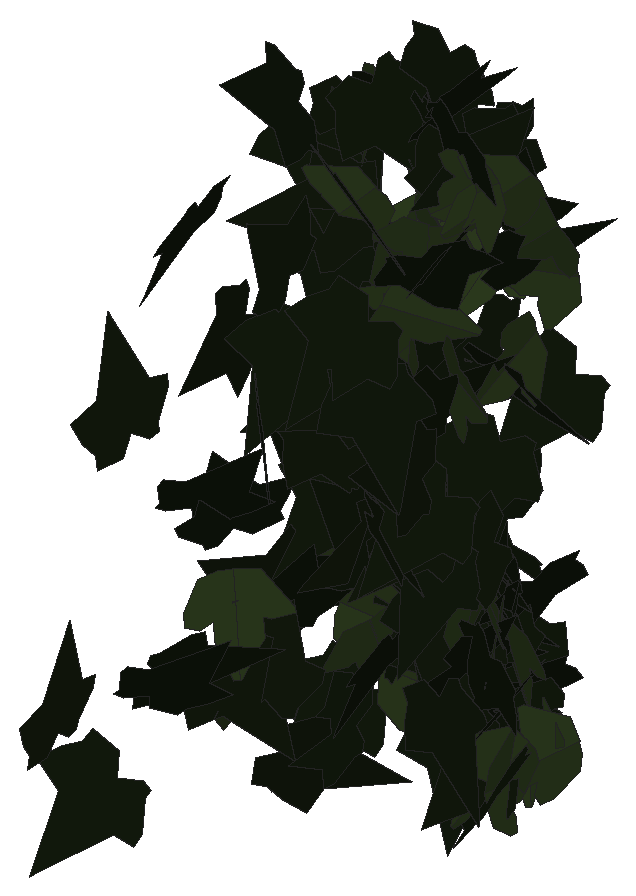
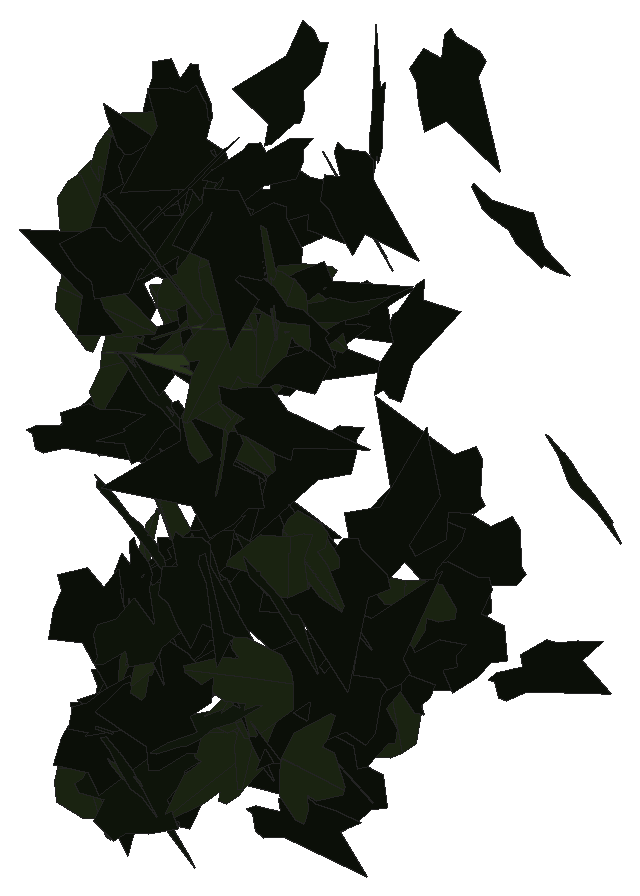
# SketchUp Ruby script. Lengths in inches.
U = 1.inch
M = Sketchup.active_model
def pt(a) = Geom::Point3d.new(a.map { |v| v * U })
def face(e, loops, mat)
  f = e.add_face(loops[0].map { |a| pt(a) })
  loops[1..].each { |l| e.add_face(l.map { |a| pt(a) }).erase! }
  f.material = f.back_material = mat if mat
  f
end
# faces: each face lists its corners as indices into pts; further lists are holes
def faces(e, pts, list, mat = nil) = list.each { |f| face(e, (f[0].is_a?(Array) ? f : [f]).map { |l| l.map { |i| pts[i] } }, mat) }
# xy, xz, yz: faces in a plane at the given z, y or x. An outline is a flat list of corners, or four numbers for a rectangle; further outlines are holes
def ring(l) = l.size == 4 ? [[l[0], l[1]], [l[2], l[1]], [l[2], l[3]], [l[0], l[3]]] : l.each_slice(2).to_a
def flat(e, list, mat, &to3) = list.each { |f| face(e, (f[0].is_a?(Array) ? f : [f]).map { |l| ring(l).map { |u, v| to3.(u, v) } }, mat) }
def xy(e, z, list, mat = nil) = flat(e, list, mat) { |x, y| [x, y, z] }
def xz(e, y, list, mat = nil) = flat(e, list, mat) { |x, z| [x, y, z] }
def yz(e, x, list, mat = nil) = flat(e, list, mat) { |y, z| [x, y, z] }
def lines(e, pts, list) = list.each { |a, b| e.add_line(pt(pts[a]), pt(pts[b])) }
# prism: a flat outline (further loops are holes) pulled along v
def prism(e, loops, v, mat = nil)
  f = face(e, loops, mat); d = Geom::Vector3d.new(v.map { |x| x * U })
  f.pushpull(f.normal.samedirection?(d) ? d.length : -d.length)
end
def box(e, o, s, mat = nil) = prism(e, [[o, [o[0] + s[0], o[1], o[2]], [o[0] + s[0], o[1] + s[1], o[2]], [o[0], o[1] + s[1], o[2]]]], [0, 0, s[2]], mat)
def at(x, y, z, deg = 0) = Geom::Transformation.translation(pt([x, y, z])) * Geom::Transformation.rotation(ORIGIN, Z_AXIS, deg.degrees)
def axes(o, x, y, z) = Geom::Transformation.new([*x, 0, *y, 0, *z, 0, *pt(o).to_a, 1])
def part(name) = M.definitions.add(name)
# library, detail: a bought-in or finely detailed component or shape, given as its bounding box
def library(name, o, s) = part(name).tap { |d| box(d.entities, o, s) }
def detail(e, o, s) = box(e.add_group.entities, o, s)
def put(e, d, t, mat = nil) = e.add_instance(d, t).tap { |i| i.material = mat if mat }
def group(e, t, mat = nil) = e.add_group.tap { |g| g.transformation = t; g.material = mat if mat }.entities
root = M.entities
M.materials.add("efeu1").color = [18, 25, 13]
M.materials.add("efeu2").color = [43, 57, 29]
c1 = part("ivyleaf_9")
p = [[1.54,2.16,1.25],[1.36,2.04,1.19],[-0.21,0.99,0.68],[-0.71,1.11,0.82],[-0.85,0.86,0.67],[-0.8,0.17,0.21],
  [-0.9,-0.01,0.1],[-0.67,-0.16,-0.02],[-0.08,-0.08,-0.05],[-0.03,-0.6,-0.4],[0.65,-0.88,-0.66],[0.83,-0.6,-0.49],
  [1.29,-0.42,-0.43],[1.8125,-0.07,-0.26],[1.21,0.44,0.15]]
faces(c1.entities,p,[[0,1,2,3,4,5,6,7,8,9,10,11,12,13,14]],"efeu1")
c2 = part("ivyleaf_10")
p = [[0,0.5,-0.03],[-0.0625,2.02,-0.43],[-0.19,2.01,-0.46],[-0.54,1.05,-0.29],[-0.52,0.625,-0.18],[-0.83,0.76,-0.28],
  [-1.16,0.64,-0.33],[-1.15,0.33,-0.24],[-0.77,-0.39,0.02],[-0.3,-0.51,0.16],[0.04,-0.48,0.23],[-0.02,2.01,-0.4375],
  [-0.06,2.01,-0.43],[0.04,-0.49,0.23],[0.67,-0.49,0.14],[1.38,0.36,-0.2],[1.375,0.51,-0.24],[0.81,0.65,-0.19],
  [0.62,0.59,-0.15],[0.6,1.09,-0.28],[0.5,1.23,-0.31]]
faces(c2.entities,p,[[0,1,2,3,4,5,6,7,8,9,10],[11,12,0,13,14,15,16,17,18,19,20]],"efeu2")
put(root,c1,axes([49.99,215.57,235.71],[-0.39967,0.22054,-0.20402],[-0.18022,0.09569,0.45647],[0.24039,0.43841,0.003]))
put(root,c1,axes([52.22,216.5,239.71],[-0.02606,0.03411,0.49815],[0.07343,-0.49315,0.0376],[0.49389,0.07512,0.02069]))
put(root,c1,axes([50.27,216.52,239.3],[-0.47515,0.08384,-0.13118],[-0.13302,0.00028,0.48198],[0.08089,0.49292,0.02204]))
put(root,c1,axes([49.53,217.14,234.17],[-0.31074,-0.35872,0.15736],[-0.10655,-0.11589,-0.47457],[0.37695,-0.32847,-0.00442]))
put(root,c1,axes([50.48,217.46,241.78],[-0.23217,0.35561,-0.26389],[0.13647,-0.226,-0.42462],[-0.42127,-0.2692,0.00789]))
put(root,c1,axes([49.88,217.44,235.3],[0.37642,0.32647,-0.04159],[0.02869,0.03039,0.49825],[0.32785,-0.37749,0.00415]))
put(root,c1,axes([49.58,218.01,235.21],[0.02408,0.29514,-0.40288],[0.03938,0.40097,0.29609],[0.49787,-0.04599,-0.00394]))
put(root,c1,axes([51.875,218.76,240.21],[-0.40406,-0.29221,0.03674],[-0.03289,-0.01721,-0.49862],[0.29267,-0.40536,-0.00532]))
put(root,c1,axes([52.09,218.73,239.49],[-0.02694,-0.47008,-0.16822],[0.03156,0.16653,-0.4704],[0.49828,-0.03596,0.0207]))
put(root,c1,axes([49.41,218.78,237],[0.38796,0.31541,0.00014],[-0.00169,0.00186,0.49999],[0.31541,-0.38796,0.0025]))
put(root,c1,axes([51.34,218.98,241.81],[0.31594,-0.31123,0.23091],[0.16229,-0.16428,-0.44348],[0.35191,0.35517,-0.00279]))
put(root,c1,axes([50.64,219.21,239.34],[-0.27085,-0.41475,0.06801],[-0.03151,-0.06064,-0.49531],[0.4191,-0.27259,0.00671]))
put(root,c1,axes([49.67,219.32,239.28],[0.00942,-0.16959,-0.47027],[0.31624,-0.36226,0.13697],[-0.38718,-0.30001,0.10044]))
put(root,c1,axes([50.76,218.77,240.5],[-0.16989,0.28729,0.37229],[-0.19955,0.31439,-0.33367],[-0.42581,-0.26196,0.00784]))
put(root,c2,axes([49.76,219.04,235.87],[0.407,0.28424,0.05961],[0.05015,0.03231,-0.49643],[-0.28607,0.41007,-0.00221]))
put(root,c1,axes([49.73,218.95,235.04],[0.03855,-0.32128,-0.38117],[0.01394,0.38285,-0.32129],[0.49832,0.01415,0.03848]))
put(root,c1,axes([52.12,219.47,238],[-0.06064,-0.06194,0.49243],[-0.20002,-0.45097,-0.08135],[0.45422,-0.20686,0.02991]))
put(root,c1,axes([49.55,219.3125,236.56],[0.30021,0.20075,0.34579],[-0.28282,-0.19905,0.3611],[0.28264,-0.41241,-0.00596]))
put(root,c2,axes([49.65,219.38,234.29],[0.02323,-0.49628,-0.05623],[0.00614,-0.056,0.49682],[-0.49942,-0.02378,0.0035]))
put(root,c1,axes([50.09,219.21,234.6],[-0.45453,0.0486,0.20258],[0.20123,-0.02344,0.45712],[0.05393,0.49708,0.00175]))
put(root,c1,axes([51.67,219.27,237.35],[0.41217,-0.17687,-0.22098],[-0.18981,0.11686,-0.44757],[0.20997,0.45284,0.02919]))
put(root,c1,axes([51,219.74,238.76],[-0.32371,-0.22221,0.30957],[-0.26412,-0.16196,-0.39244],[0.27468,-0.4176,-0.01253]))
put(root,c1,axes([51.67,219.51,235.67],[-0.21928,0.35771,-0.27195],[0.12805,-0.24032,-0.41935],[-0.43072,-0.25355,0.01378]))
put(root,c1,axes([52.16,219.8,237.59],[-0.36068,-0.33052,0.10327],[-0.07652,-0.06935,-0.48922],[0.33772,-0.36871,-0.00056]))
put(root,c1,axes([52.24,219.77,236.86],[-0.42698,-0.17845,-0.18931],[0.19423,0.02341,-0.46014],[0.17309,-0.46648,0.04933]))
put(root,c1,axes([49.86,219.67,235.33],[0.35674,0.31707,0.14902],[-0.11277,-0.09743,0.47727],[0.33169,-0.37413,0.00199]))
put(root,c1,axes([49.65,220,235.33],[0.05053,0.04046,0.49579],[-0.36123,-0.33963,0.06453],[0.34199,-0.36471,-0.00509]))
put(root,c1,axes([50.97,219.68,234.27],[-0.4208,0.24404,0.11564],[-0.10703,0.04586,-0.48625],[-0.24793,-0.43398,0.01364]))
put(root,c1,axes([50.17,219.48,233.73],[0.11932,0.13314,-0.46694],[0.22307,0.41205,0.1745],[0.43128,-0.24997,0.03893]))
put(root,c1,axes([51.97,219.96,237.24],[-0.49563,-0.06499,0.01127],[-0.01088,-0.00367,-0.49987],[0.06505,-0.49574,0.00222]))
put(root,c1,axes([51.45,220.13,236.82],[-0.07828,-0.03733,-0.49242],[0.01006,-0.49859,0.0362],[-0.49373,-0.00424,0.07881]))
put(root,c1,axes([51.17,219.64,236.79],[-0.28381,0.04697,-0.40896],[-0.41137,-0.01428,0.28385],[0.01498,0.49758,0.04675]))
put(root,c1,axes([52.07,219.93,234.85],[0.17337,-0.45792,-0.10124],[-0.03661,0.09439,-0.48964],[0.46755,0.17719,-0.0008]))
put(root,c1,axes([52.73,219.98,237.13],[-0.49394,0.07522,-0.01909],[0.01888,-0.00279,-0.49964],[-0.07527,-0.4943,-0.00008]))
put(root,c2,axes([52.0625,220.16,238.91],[-0.07368,-0.00952,0.49445],[0.47229,-0.14961,0.0675],[0.14666,0.477,0.03104]))
put(root,c1,axes([51.78,219.67,238.54],[0.1472,0.037,0.47641],[0.35605,0.32397,-0.13517],[-0.31869,0.37904,0.06903]))
put(root,c1,axes([50.36,219.93,237.98],[0.06698,-0.32711,-0.37217],[-0.04897,0.36935,-0.33344],[0.49307,0.08112,0.01744]))
put(root,c1,axes([49.59,219.68,234.74],[0.0962,0.1016,0.48002],[0.25664,0.40649,-0.13747],[-0.41819,0.27284,0.02606]))
put(root,c1,axes([49.73,220.2,241.74],[-0.11921,0.07273,-0.4801],[-0.46417,-0.16227,0.09067],[-0.14262,0.46731,0.1062]))
put(root,c1,axes([51.73,220.04,240.45],[0.26999,0.41183,-0.08662],[-0.05092,-0.07019,-0.49242],[-0.41775,0.27472,0.00404]))
put(root,c1,axes([52.59,220.16,235.5],[0.21252,0.03055,-0.45156],[-0.44708,-0.06345,-0.2147],[-0.07042,0.49502,0.00034]))
put(root,c1,axes([52.73,220.09,233.81],[-0.20504,0.4481,0.08467],[-0.05113,0.06966,-0.49248],[-0.45315,-0.21061,0.01725]))
put(root,c1,axes([52.09,220.21,242.14],[0.29541,0.04984,-0.40031],[-0.39674,-0.05391,-0.29949],[-0.07302,0.49458,0.0077]))
put(root,c2,axes([52.32,220.34,241.45],[0.31265,-0.09073,-0.37949],[-0.35328,0.14062,-0.32468],[0.16565,0.47116,0.02382]))
put(root,c1,axes([52.11,220.81,233.84],[-0.18336,-0.35735,0.29779],[-0.08563,-0.28869,-0.39915],[0.45722,-0.19737,0.04467]))
put(root,c1,axes([51.96,220.24,240.62],[-0.15813,0.47417,0.01274],[-0.00506,0.01174,-0.49984],[-0.47431,-0.1582,0.00108]))
put(root,c1,axes([52.25,220.71,237.91],[-0.28018,-0.41409,-0.00499],[0.00341,0.00372,-0.49997],[0.41411,-0.2802,0.00074]))
put(root,c2,axes([52.5,220.7,241.41],[-0.17605,-0.2401,0.40169],[-0.2174,-0.3381,-0.29737],[0.41442,-0.27936,0.01465]))
put(root,c1,axes([50.11,220.76,240.19],[-0.25711,-0.10221,0.41647],[-0.36286,-0.20693,-0.27479],[0.22853,-0.44355,0.03223]))
put(root,c1,axes([50.125,220.69,236.66],[-0.47589,-0.15337,-0.00221],[0.00194,0.0012,-0.49999],[0.15337,-0.4759,-0.00054]))
put(root,c2,axes([51.2,220.27,239.54],[-0.17072,-0.16609,-0.43962],[0.34642,0.2716,-0.23713],[0.31757,-0.38555,0.02233]))
put(root,c2,axes([52.33,220.87,233.82],[-0.11496,-0.28818,0.39209],[-0.03267,-0.3974,-0.30167],[0.48551,-0.09497,0.07254]))
put(root,c2,axes([52.43,220.32,236.26],[-0.27092,0.28598,0.30793],[-0.22,0.21564,-0.39383],[-0.35805,-0.34888,0.00899]))
put(root,c1,axes([49.81,220.82,239.75],[-0.06269,-0.49605,0.00153],[-0.00055,-0.00147,-0.5],[0.49605,-0.06269,-0.00036]))
put(root,c2,axes([50.1875,220.8,240.38],[-0.26344,-0.19099,0.37963],[-0.23738,-0.30435,-0.31784],[0.35249,-0.3477,0.06969]))
put(root,c1,axes([51.58,220.71,235.31],[-0.29826,-0.29276,-0.27447],[0.19674,0.19138,-0.41793],[0.34977,-0.3573,0.00103]))
put(root,c2,axes([51.91,220.72,235.92],[-0.05525,-0.49582,0.03325],[-0.00195,-0.03324,-0.49889],[0.49693,-0.05525,0.00174]))
put(root,c1,axes([49.54,220.35,235.4375],[0.3697,0.30601,0.1403],[0.10811,0.08943,-0.47991],[-0.31881,0.38518,-0.00004]))
put(root,c1,axes([49.97,220.96,233.8],[-0.44796,-0.22133,0.01858],[-0.01694,-0.00766,-0.49965],[0.22146,-0.44828,-0.00064]))
put(root,c1,axes([51.42,221.11,236.68],[-0.24668,-0.35096,0.25685],[-0.11779,-0.23034,-0.42786],[0.41866,-0.2716,0.03096]))
put(root,c2,axes([50.51,220.65,234.93],[-0.20878,-0.41964,-0.17411],[0.07887,0.15523,-0.4687],[0.44743,-0.22317,0.00138]))
put(root,c1,axes([51.93,220.37,235.1],[0.21299,0.32313,0.31658],[0.1835,0.25811,-0.38692],[-0.41347,0.28101,-0.00864]))
put(root,c1,axes([50.51,220.67,241.98],[0.11021,-0.34893,-0.34074],[-0.01275,0.34715,-0.35962],[0.48754,0.08795,0.06762]))
put(root,c2,axes([51.24,220.77,240.23],[-0.45605,-0.19339,0.06796],[-0.05787,-0.03755,-0.49522],[0.19664,-0.45956,0.01187]))
put(root,c1,axes([51.7,220.68,241.02],[-0.22339,0.05507,0.44392],[0.43173,-0.10332,0.23008],[0.11707,0.4861,-0.00139]))
put(root,c1,axes([51.22,221.12,235.26],[-0.10541,-0.48705,0.04091],[0.01583,-0.04523,-0.4977],[0.48851,-0.10363,0.02495]))
put(root,c2,axes([52.46,220.49,233.61],[-0.05768,0.09711,0.48708],[-0.22536,0.43185,-0.11278],[-0.44259,-0.23255,-0.00605]))
put(root,c1,axes([51.4,221.15,233.72],[-0.07171,-0.49475,0.00913],[-0.01459,-0.0071,-0.49974],[0.49462,-0.07194,-0.01342]))
put(root,c2,axes([52.25,221.26,238.97],[0.04398,0.17369,-0.46679],[-0.09293,-0.45752,-0.179],[-0.48932,0.1025,-0.00796]))
put(root,c2,axes([51.68,221.01,237.27],[0.41931,-0.26637,-0.0568],[-0.04962,0.02781,-0.49675],[0.26779,0.42223,-0.00312]))
put(root,c1,axes([51.02,221.07,236.52],[0.34371,-0.24867,0.26463],[0.21841,-0.14954,-0.42419],[0.29011,0.40719,0.00583]))
put(root,c1,axes([49.2,221.3,240.6],[-0.11428,-0.48377,0.05391],[0.26843,-0.10882,-0.40756],[0.40606,-0.06421,0.28459]))
put(root,c2,axes([51.99,221.24,235.51],[-0.12297,0.29772,-0.38241],[0.03058,-0.38898,-0.31267],[-0.48368,-0.10028,0.07746]))
put(root,c1,axes([51.89,221.39,241.45],[-0.01754,-0.12228,-0.4845],[0.12065,-0.47149,0.11463],[-0.48491,-0.11289,0.04605]))
put(root,c2,axes([50.18,220.82,234.96],[0.11398,0.08462,0.47942],[0.37235,0.30206,-0.14184],[-0.31363,0.38936,0.00585]))
put(root,c1,axes([49.4,220.93,237.22],[0.17344,0.3814,-0.27286],[-0.14157,-0.23477,-0.41814],[-0.44707,0.22231,0.02655]))
put(root,c1,axes([52.28,220.88,234.52],[-0.19154,0.4615,-0.0181],[-0.00003,-0.0196,-0.49962],[-0.46186,-0.19139,0.00754]))
put(root,c2,axes([52.83,220.99,240.81],[-0.31818,-0.00999,0.38556],[-0.38567,0.00289,-0.3182],[0.00413,-0.49989,-0.00955]))
put(root,c2,axes([50.69,221.26,238.95],[-0.24846,-0.30811,0.30552],[-0.17595,-0.25027,-0.39548],[0.39663,-0.30403,0.01594]))
put(root,c2,axes([52.24,221,235.36],[-0.44825,0.21565,0.05065],[-0.0455,0.02227,-0.49743],[-0.2168,-0.45055,-0.00034]))
put(root,c1,axes([50.69,220.89,234.71],[-0.10705,0.19565,0.44751],[-0.25026,0.37144,-0.22226],[-0.41941,-0.27157,0.0184]))
put(root,c1,axes([51.36,220.72,241.91],[0.18891,0.26978,0.37621],[0.12401,0.36199,-0.32185],[-0.44602,0.2149,0.06985]))
put(root,c1,axes([51.15,221.13,236.32],[0.06022,0.01113,-0.49624],[0.44924,0.21136,0.05926],[0.21109,-0.45299,0.01545]))
put(root,c2,axes([52.5,221.5,233.69],[-0.11387,-0.07316,0.48133],[-0.10927,-0.47787,-0.09849],[0.47444,-0.12762,0.09284]))
put(root,c2,axes([51.04,220.95,240.52],[-0.18099,0.22778,-0.40665],[-0.29276,0.28388,0.28931],[0.36267,0.34283,0.03062]))
put(root,c1,axes([52.03,221.08,234.92],[-0.09378,0.16488,0.46262],[-0.41886,0.21907,-0.16299],[-0.25645,-0.41811,0.09704]))
put(root,c1,axes([51.76,221.1,238.6],[0.45767,-0.1096,0.16888],[0.16748,-0.02549,-0.47043],[0.11173,0.48717,0.01338]))
put(root,c1,axes([51.89,221.16,238.9],[-0.39488,0.29635,0.07903],[-0.07741,0.02836,-0.49316],[-0.29678,-0.40171,0.02349]))
put(root,c1,axes([51.43,221.34,236.13],[0.30121,-0.38264,0.1134],[0.06861,-0.0903,-0.48697],[0.39315,0.30892,-0.00189]))
put(root,c2,axes([50.8,221.58,240.03],[-0.45108,-0.18415,0.11233],[0.16931,-0.46359,-0.08012],[0.13366,-0.03424,0.48059]))
put(root,c1,axes([52.16,220.99,236.87],[-0.07275,0.32024,0.37703],[-0.2514,0.30427,-0.30695],[-0.42604,-0.23423,0.11674]))
put(root,c1,axes([51.79,221.33,240.45],[0.42693,0.21868,0.14111],[-0.13572,-0.04424,0.47919],[0.22206,-0.44746,0.02158]))
put(root,c2,axes([50.68,220.98,234.25],[0.04493,0.26426,0.42207],[0.09304,0.41187,-0.26778],[-0.48921,0.1026,-0.01216]))
put(root,c2,axes([49.97,221.24,235.63],[-0.04494,-0.00982,-0.49788],[0.49646,0.0381,-0.04556],[0.03884,-0.49845,0.00633]))
put(root,c2,axes([49.59,221.19,237.52],[0.18415,-0.10666,-0.45245],[-0.3775,0.24968,-0.2125],[0.27127,0.41986,0.01143]))
put(root,c1,axes([52.01,221.18,236.32],[0.04782,0.04377,-0.49578],[-0.49765,-0.00319,-0.04829],[-0.00739,0.49807,0.04326]))
put(root,c1,axes([52.36,221.23,235.9375],[-0.02203,0.47687,-0.14869],[0.02105,-0.14781,-0.47719],[-0.49907,-0.02729,-0.01357]))
put(root,c1,axes([51.98,221.11,240.03],[0.21028,0.39541,-0.22234],[0.0979,0.19974,0.4478],[0.44294,-0.23186,0.00658]))
put(root,c1,axes([50.08,221.45,239.08],[-0.31377,0.07854,0.38129],[-0.37955,0.04717,-0.32206],[-0.08656,-0.49154,0.03002]))
put(root,c1,axes([50.03,221.1875,237.05],[-0.25485,0.38961,0.18237],[-0.11602,0.14187,-0.4652],[-0.41424,-0.27943,0.0181]))
put(root,c1,axes([50.79,221.375,241.52],[0.38465,-0.31065,-0.07445],[-0.05414,0.05144,-0.49439],[0.31482,0.3884,0.00593]))
put(root,c1,axes([52.11,221.73,234.46],[-0.20431,-0.13829,0.4349],[-0.35381,-0.25295,-0.24665],[0.28823,-0.40853,0.0055]))
put(root,c2,axes([49.16,221.74,235.04],[0.03187,-0.30014,0.39862],[0.09461,-0.38855,-0.30013],[0.48993,0.09456,0.03203]))
put(root,c2,axes([49.54,221.41,237.55],[0.36359,0.34281,0.01686],[0.01044,0.01351,-0.49971],[-0.34307,0.36373,0.00267]))
put(root,c2,axes([50.61,221.1,238.51],[-0.02606,0.29126,-0.40557],[-0.12327,0.3898,0.28785],[0.48386,0.115,0.05149]))
put(root,c1,axes([50.77,221.125,236.55],[-0.19411,0.0936,-0.45118],[-0.39814,0.21239,0.21535],[0.23196,0.44287,-0.00793]))
put(root,c2,axes([50.53,221.26,239.84],[-0.16766,-0.36286,-0.30037],[0.14112,0.2655,-0.3995],[0.44942,-0.21873,0.01339]))
put(root,c2,axes([51.36,221.83,239.59],[-0.49887,-0.02712,0.01989],[0.02293,-0.49059,-0.09379],[0.0246,-0.09267,0.49072]))
put(root,c1,axes([50.74,221.75,241.99],[0.05692,-0.48195,0.12035],[0.04855,-0.11516,-0.48413],[0.49437,0.0668,0.03369]))
put(root,c2,axes([49.92,221.36,241.28],[0.23397,-0.32802,-0.29608],[-0.14445,0.25984,-0.40201],[0.41761,0.27365,0.02683]))
put(root,c1,axes([50.42,221.72,235.09],[0.05387,-0.4925,0.06739],[0.22314,-0.03661,-0.44595],[0.44419,0.07812,0.21585]))
put(root,c2,axes([52.48,221.51,239.88],[0.09723,0.02144,-0.48999],[-0.48603,0.07117,-0.09333],[0.06574,0.49444,0.03469]))
put(root,c1,axes([51.48,221.9,235.85],[-0.31185,-0.22356,0.32058],[0.16586,-0.44706,-0.15042],[0.35389,0.01252,0.35299]))
put(root,c2,axes([51.95,221.59,233.89],[0.47624,-0.04664,0.14499],[0.14629,0.00764,-0.47806],[0.04238,0.49776,0.02092]))
put(root,c2,axes([51.64,221.23,235.23],[0.13442,-0.10334,0.47038],[-0.2787,0.38158,0.16347],[-0.39276,-0.30613,0.04498]))
put(root,c1,axes([51.73,221.92,233.8125],[-0.49284,-0.08434,-0.00031],[0.08243,-0.48133,-0.10737],[0.01782,-0.10588,0.48834]))
put(root,c1,axes([50.15,221.38,241.59],[0.31928,0.33268,-0.19335],[-0.14517,-0.12853,-0.46087],[-0.35636,0.35043,0.01452]))
put(root,c1,axes([52.4,221.86,238.36],[-0.37433,-0.31689,0.09723],[-0.05923,-0.08036,-0.48993],[0.32614,-0.37831,0.02262]))
put(root,c1,axes([52.01,221.42,234.42],[0.05842,0.47906,-0.13073],[-0.01519,-0.12984,-0.48261],[-0.49634,0.06036,-0.00062]))
put(root,c1,axes([50.5,221.33,238.27],[0.13287,0.0822,-0.47496],[0.19702,0.44038,0.13134],[0.43992,-0.22206,0.08463]))
put(root,c1,axes([51.8125,221.5625,234.12],[-0.3909,0.30786,0.04916],[-0.03807,0.03112,-0.49758],[-0.30943,-0.39275,-0.00089]))
put(root,c1,axes([49.29,221.78,240.9375],[-0.20975,-0.21242,-0.4011],[0.39506,0.13209,-0.27655],[0.22345,-0.43293,0.11243]))
put(root,c2,axes([49.5,221.58,240.89],[-0.47836,0.13764,-0.0472],[0.04443,-0.01629,-0.49776],[-0.13856,-0.48041,0.00336]))
put(root,c1,axes([51.78,221.63,241.19],[-0.42896,0.25166,0.05154],[-0.04366,0.02744,-0.49733],[-0.25315,-0.43118,-0.00157]))
put(root,c1,axes([50.84,221.67,235.08],[0.33817,-0.12266,0.34727],[0.32531,-0.12155,-0.35972],[0.17267,0.46923,-0.0024]))
put(root,c1,axes([50.72,221.89,237.09],[-0.31076,0.18545,-0.34502],[0.21157,-0.29117,-0.34707],[-0.32965,-0.3617,0.1025]))
